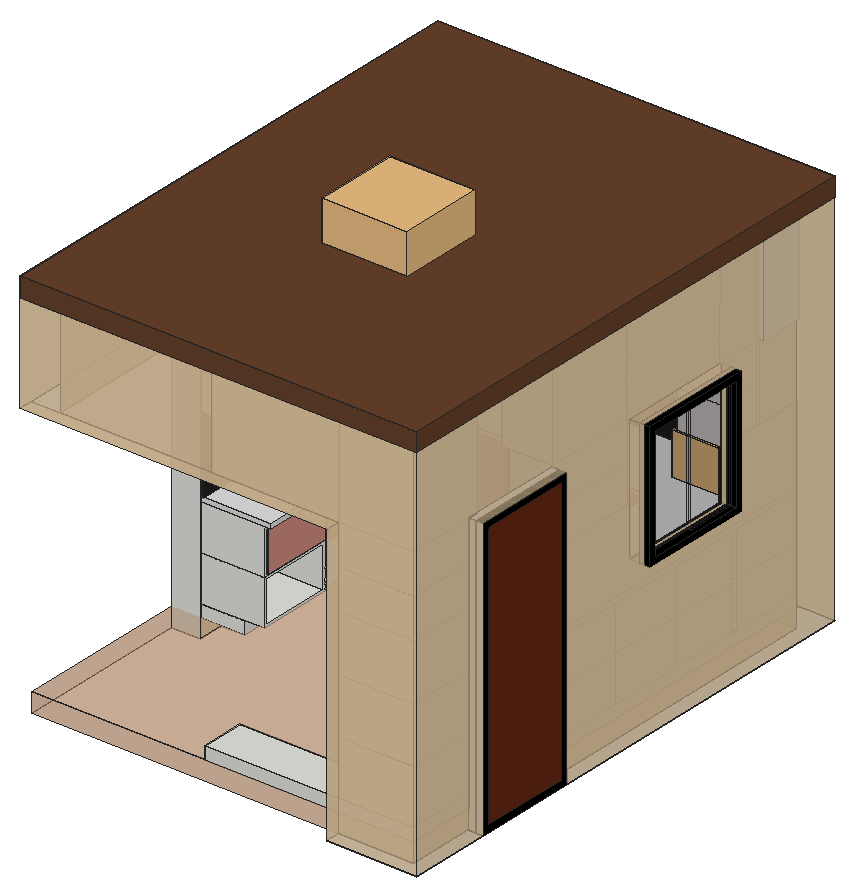
# SketchUp Ruby script. Lengths in inches.
U = 1.inch
M = Sketchup.active_model
def pt(a) = Geom::Point3d.new(a.map { |v| v * U })
def face(e, loops, mat)
  f = e.add_face(loops[0].map { |a| pt(a) })
  loops[1..].each { |l| e.add_face(l.map { |a| pt(a) }).erase! }
  f.material = f.back_material = mat if mat
  f
end
# faces: each face lists its corners as indices into pts; further lists are holes
def faces(e, pts, list, mat = nil) = list.each { |f| face(e, (f[0].is_a?(Array) ? f : [f]).map { |l| l.map { |i| pts[i] } }, mat) }
# xy, xz, yz: faces in a plane at the given z, y or x. An outline is a flat list of corners, or four numbers for a rectangle; further outlines are holes
def ring(l) = l.size == 4 ? [[l[0], l[1]], [l[2], l[1]], [l[2], l[3]], [l[0], l[3]]] : l.each_slice(2).to_a
def flat(e, list, mat, &to3) = list.each { |f| face(e, (f[0].is_a?(Array) ? f : [f]).map { |l| ring(l).map { |u, v| to3.(u, v) } }, mat) }
def xy(e, z, list, mat = nil) = flat(e, list, mat) { |x, y| [x, y, z] }
def xz(e, y, list, mat = nil) = flat(e, list, mat) { |x, z| [x, y, z] }
def yz(e, x, list, mat = nil) = flat(e, list, mat) { |y, z| [x, y, z] }
def lines(e, pts, list) = list.each { |a, b| e.add_line(pt(pts[a]), pt(pts[b])) }
# prism: a flat outline (further loops are holes) pulled along v
def prism(e, loops, v, mat = nil)
  f = face(e, loops, mat); d = Geom::Vector3d.new(v.map { |x| x * U })
  f.pushpull(f.normal.samedirection?(d) ? d.length : -d.length)
end
def box(e, o, s, mat = nil) = prism(e, [[o, [o[0] + s[0], o[1], o[2]], [o[0] + s[0], o[1] + s[1], o[2]], [o[0], o[1] + s[1], o[2]]]], [0, 0, s[2]], mat)
def at(x, y, z, deg = 0) = Geom::Transformation.translation(pt([x, y, z])) * Geom::Transformation.rotation(ORIGIN, Z_AXIS, deg.degrees)
def axes(o, x, y, z) = Geom::Transformation.new([*x, 0, *y, 0, *z, 0, *pt(o).to_a, 1])
def part(name) = M.definitions.add(name)
# library, detail: a bought-in or finely detailed component or shape, given as its bounding box
def library(name, o, s) = part(name).tap { |d| box(d.entities, o, s) }
def detail(e, o, s) = box(e.add_group.entities, o, s)
def put(e, d, t, mat = nil) = e.add_instance(d, t).tap { |i| i.material = mat if mat }
def group(e, t, mat = nil) = e.add_group.tap { |g| g.transformation = t; g.material = mat if mat }.entities
root = M.entities
M.materials.add("BEIGE FOR CUPBOARDS").color = [205, 139, 125]
M.materials.add("Chocolate White WALL PAINT").color = [230, 202, 161]
M.materials["Chocolate White WALL PAINT"].alpha = 0.75
M.materials.add("GLASS").color = [0, 0, 0]
M.materials["GLASS"].alpha = 0.1
M.materials.add("METAL").color = [0, 0, 0]
M.materials.add("Marble Black 100cm").color = [32, 32, 32]
M.materials.add("Marble White SSS 100cm").color = [222, 222, 222]
M.materials.add("Onyx 100cm").color = [192, 149, 115]
M.materials["Onyx 100cm"].alpha = 0.47
M.materials.add("Roof Ceramic 22-10 200cm").color = [102, 65, 42]
M.materials.add("WHITE  FOR CUPBOARDS").color = [218, 213, 212]
M.materials.add("Wood Dark 02 100cm").color = [99, 39, 19]
M.materials["Wood Dark 02 100cm"].alpha = 0.97
c1 = library("Cutlery Box 145 009",[-8.61,-2.8,0],[17.18,6.16,8.82])
c2 = library("Spice Stand 145 027",[-6.18,-5.51,0],[12.36,11.02,14.15])
c3 = library("Breakfast Meal Set 145 006",[-7.73,-8.125,0],[15.46,19.06,8.53])
c4 = library("Kitchen Props 134 014",[-15.6875,-7.04,0],[31.37,14.09,12.97])
c5 = library("Sphere Light",[-13.29,-13.29,-13.29],[26.58,26.58,26.58])
c6 = library("Spot Light",[-5.1,-5.1,-11.05],[10.2,10.2,11.05])
c7 = library("Spot Light\#1",[-5.1,-5.1,-11.05],[10.2,10.2,11.05])
c8 = library("Spot Light\#2",[-5.1,-5.1,-11.05],[10.2,10.2,11.05])
c9 = library("Spot Light\#3",[-5.1,-5.1,-11.05],[10.2,10.2,11.05])
c10 = part("Group\#20")
xy(c10.entities,0,[[0,-2.26,23.62,21.36]])
xy(c10.entities,0.81,[[0,-1.45,22.05,20.56]])
xy(c10.entities,13.37,[[0,-1.45,22.05,20.56]])
xy(c10.entities,14.17,[[0,-2.26,23.62,21.36]])
xz(c10.entities,-2.26,[[0,0,23.62,14.17]])
xz(c10.entities,-1.45,[[0,0.81,22.05,13.37]])
xz(c10.entities,20.56,[[0,0.81,22.05,13.37]])
xz(c10.entities,21.36,[[0,0,23.62,14.17]])
yz(c10.entities,0,[[[-2.16,0.1,21.26,14.07],[-1.45,0.81,20.56,13.37]]])
yz(c10.entities,22.05,[[-1.45,0.81,20.56,13.37]])
yz(c10.entities,23.62,[[-2.26,0,21.36,14.17]])
c11 = part("Group\#23")
box(c11.entities,[-0.71,0,0],[0.71,22.01,12.56])
c12 = part("Group\#40")
xy(c12.entities,0,[[0,-1.97,19.78,21.65]])
xy(c12.entities,0.71,[[4.04,-1.26,19.78,20.94]])
xy(c12.entities,13.46,[[4.04,-1.26,19.78,20.94]])
xy(c12.entities,14.17,[[0,-1.97,19.78,21.65]])
xz(c12.entities,-1.97,[[0,0,19.78,14.17]])
xz(c12.entities,-1.26,[[4.04,0.71,19.78,13.46]])
xz(c12.entities,20.94,[[4.04,0.71,19.78,13.46]])
xz(c12.entities,21.65,[[0,0,19.78,14.17]])
yz(c12.entities,0,[[-1.97,0,21.65,14.17]])
yz(c12.entities,4.04,[[-1.26,0.71,20.94,13.46]])
yz(c12.entities,19.78,[[[-1.87,0.1,21.56,14.07],[-1.26,0.71,20.94,13.46]]])
c13 = part("Group\#43")
box(c13.entities,[0,0,0],[0.71,22.01,12.56])
c14 = part("Group\#24")
box(c14.entities,[0,-2.26,0],[23.62,23.62,14.17])
c15 = part("Group\#82")
box(c15.entities,[0,-0.71,0],[13.35,0.71,10.2])
c16 = part("Group\#62")
box(c16.entities,[-0.71,0,0],[0.71,17.3,27.91])
c17 = part("Group\#79")
box(c17.entities,[0,1,-0.35],[6.26,10.8125,0.7])
c18 = part("Group\#63")
box(c18.entities,[-0.71,0,0],[0.71,13.86,28.11])
c19 = part("Group\#84")
box(c19.entities,[0,-0.71,0],[13.54,0.71,28.11])
c20 = part("Group\#92")
box(c20.entities,[0,0,0],[0.71,22.01,10.2])
c21 = part("Group\#93")
box(c21.entities,[0,0,0],[0.71,22.2,28.11])
p = [[119.24,25.58,0],[123.74,25.58,0]]
lines(root,p,[[0,1]])
put(root,c1,at(19.45,148.53,39.86))
put(root,c2,at(16.11,131.18,39.85,90))
put(root,c3,at(21.28,114.77,39.86,-180))
put(root,c4,axes([105.33,146.65,39.86],[0.82,0,0],[0,1.17,0],[0,0,1]))
put(root,c5,at(60.16,72.25,123.27))
put(root,c6,at(30.14,28.18,118.19))
put(root,c7,at(93.57,127.28,118.19))
put(root,c8,at(29.38,127.67,118.19))
put(root,c9,at(102.72,34.74,118.19))
g1 = group(root,at(0,0,0))
g2 = group(g1,at(0,0,0))
g3 = group(g2,at(0,0,0))
g4 = group(g3,at(9,106.47,24.11))
xy(g4,0,[[0,0,19.78,21.65]])
xy(g4,0.81,[[4.04,0.81,19.78,20.85]])
xy(g4,13.37,[[4.04,0.81,19.78,20.85]])
xy(g4,14.17,[[0,0,19.78,21.65]])
xz(g4,0,[[0,0,19.78,14.17]])
xz(g4,0.81,[[4.04,0.81,19.78,13.37]])
xz(g4,20.85,[[4.04,0.81,19.78,13.37]])
xz(g4,21.65,[[0,0,19.78,14.17]])
yz(g4,0,[[0,0,21.65,14.17]])
yz(g4,4.04,[[0.81,0.81,20.85,13.37]])
yz(g4,19.78,[[[0.1,0.1,21.56,14.07],[0.81,0.81,20.85,13.37]]])
g5 = group(g3,at(9,4.5,9.9375))
put(g5,c10,at(86.61,56.98,0))
g6 = group(g5,at(86.61,56.98,14.17))
xy(g6,0,[[0,-2.26,23.62,21.36]])
xy(g6,0.81,[[0,-1.45,22.05,20.56]])
xy(g6,13.37,[[0,-1.45,22.05,20.56]])
xy(g6,14.17,[[0,-2.26,23.62,21.36]])
xz(g6,-2.26,[[0,0,23.62,14.17]])
xz(g6,-1.45,[[0,0.81,22.05,13.37]])
xz(g6,20.56,[[0,0.81,22.05,13.37]])
xz(g6,21.36,[[0,0,23.62,14.17]])
yz(g6,0,[[[-2.16,0.1,21.26,14.07],[-1.45,0.81,20.56,13.37]]])
yz(g6,22.05,[[-1.45,0.81,20.56,13.37]])
yz(g6,23.62,[[-2.26,0,21.36,14.17]])
put(g6,c11,at(0,-1.45,0.81),"BEIGE FOR CUPBOARDS")
g7 = group(g5,at(86.61,0,17.22),"WHITE  FOR CUPBOARDS")
xy(g7,0,[[0,0,23.62,24.56]])
xy(g7,0.71,[[0.71,4.875,22.91,24.56]])
xy(g7,16.52,[[0.71,4.875,22.91,24.56]])
xy(g7,17.22,[[0,0,23.62,24.56]])
xz(g7,0,[[0,0,23.62,17.22]])
xz(g7,4.875,[[0.71,0.71,22.91,16.52]])
xz(g7,24.56,[[[0.1,0.1,23.52,17.125],[0.71,0.71,22.91,16.52]]])
yz(g7,0,[[0,0,24.56,17.22]])
yz(g7,0.71,[[4.875,0.71,24.56,16.52]])
yz(g7,22.91,[[4.875,0.71,24.56,16.52]])
yz(g7,23.62,[[0,0,24.56,17.22]])
g8 = group(g5,at(86.61,0,0),"WHITE  FOR CUPBOARDS")
xy(g8,0,[[0,0,23.62,24.56]])
xy(g8,0.81,[[0.81,4.75,22.81,24.56]])
xy(g8,16.42,[[0.81,4.75,22.81,24.56]])
xy(g8,17.22,[[0,0,23.62,24.56]])
xz(g8,0,[[0,0,23.62,17.22]])
xz(g8,4.75,[[0.81,0.81,22.81,16.42]])
xz(g8,24.56,[[[0.1,0.1,23.52,17.125],[0.81,0.81,22.81,16.42]]])
yz(g8,0,[[0,0,24.56,17.22]])
yz(g8,0.81,[[4.75,0.81,24.56,16.42]])
yz(g8,22.81,[[4.75,0.81,24.56,16.42]])
yz(g8,23.62,[[0,0,24.56,17.22]])
g9 = group(g5,at(86.61,0,52.17),"WHITE  FOR CUPBOARDS")
xy(g9,0,[[0,0,23.62,24.56]])
xy(g9,0.81,[[0.81,4.875,22.81,24.56]])
xy(g9,11.69,[[0.81,4.875,22.81,24.56]])
xy(g9,12.5,[[0,0,23.62,24.56]])
xz(g9,0,[[0,0,23.62,12.5]])
xz(g9,4.875,[[0.81,0.81,22.81,11.69]])
xz(g9,24.56,[[[0.1,0.1,23.52,12.4],[0.81,0.81,22.81,11.69]]])
yz(g9,0,[[0,0,24.56,12.5]])
yz(g9,0.81,[[4.875,0.81,24.56,11.69]])
yz(g9,22.81,[[4.875,0.81,24.56,11.69]])
yz(g9,23.62,[[0,0,24.56,12.5]])
g10 = group(g5,at(86.61,0,77.17))
xy(g10,0,[[0,0,23.62,24.56]],"WHITE  FOR CUPBOARDS")
xy(g10,29.53,[[0,0,23.62,24.56]],"WHITE  FOR CUPBOARDS")
xz(g10,0,[[0,0,23.62,29.53]],"WHITE  FOR CUPBOARDS")
yz(g10,0,[[0,0,24.56,29.53]],"WHITE  FOR CUPBOARDS")
yz(g10,23.62,[[0,0,24.56,29.53]],"WHITE  FOR CUPBOARDS")
g11 = group(g10,at(0.1,4.875,0.1),"BEIGE FOR CUPBOARDS")
xy(g11,0.71,[[0.71,0,22.72,19.69],[0.71,19.69,22.72,20.39]])
xy(g11,28.62,[[0.71,0,22.72,19.69],[0.71,19.69,22.72,20.39]])
xz(g11,0,[[0.71,0.71,22.72,28.62]])
xz(g11,19.69,[[[0,0,23.43,29.33],[0.71,0.71,22.72,28.62]]],"WHITE  FOR CUPBOARDS")
xz(g11,20.39,[[0.71,0.71,22.72,28.62]])
yz(g11,0.71,[[0,0.71,19.69,28.62],[19.69,0.71,20.39,28.62]])
yz(g11,22.72,[[0,0.71,19.69,28.62],[19.69,0.71,20.39,28.62]])
g12 = group(g5,at(86.61,0,34.45),"WHITE  FOR CUPBOARDS")
xy(g12,0,[[0,0,23.62,24.56]])
xy(g12,0.81,[[0.81,4.875,22.81,24.56]])
xy(g12,16.91,[[0.81,4.875,22.81,24.56]])
xy(g12,17.72,[[0,0,23.62,24.56]])
xz(g12,0,[[0,0,23.62,17.72]])
xz(g12,4.875,[[0.81,0.81,22.81,16.91]])
xz(g12,24.56,[[[0.1,0.1,23.52,17.62],[0.81,0.81,22.81,16.91]]])
yz(g12,0,[[0,0,24.56,17.72]])
yz(g12,0.81,[[4.875,0.81,24.56,16.91]])
yz(g12,22.81,[[4.875,0.81,24.56,16.91]])
yz(g12,23.62,[[0,0,24.56,17.72]])
g13 = group(g5,at(62.99,0,77.17))
xy(g13,0,[[-15.75,0,23.62,24.56]],"WHITE  FOR CUPBOARDS")
xy(g13,0.81,[[-14.94,4.875,22.81,24.56]])
xy(g13,28.72,[[-14.94,4.875,22.81,24.56]])
xy(g13,29.53,[[-15.75,0,23.62,24.56]],"WHITE  FOR CUPBOARDS")
xz(g13,0,[[-15.75,0,23.62,29.53]],"WHITE  FOR CUPBOARDS")
xz(g13,4.875,[[-14.94,0.81,22.81,28.72]])
xz(g13,24.56,[[[-15.65,0.1,23.52,29.43],[-14.94,0.81,22.81,28.72]]],"WHITE  FOR CUPBOARDS")
yz(g13,-15.75,[[0,0,24.56,29.53]],"WHITE  FOR CUPBOARDS")
yz(g13,-14.94,[[4.875,0.81,24.56,28.72]])
yz(g13,22.81,[[4.875,0.81,24.56,28.72]])
yz(g13,23.62,[[0,0,24.56,29.53]],"WHITE  FOR CUPBOARDS")
g14 = group(g13,at(3.9375,24.56,0.81),"BEIGE FOR CUPBOARDS")
box(g14,[0,0,0],[18.88,0.71,27.91])
g15 = group(g13,at(-14.94,24.56,0.81),"BEIGE FOR CUPBOARDS")
box(g15,[0,0,0],[18.88,0.71,27.91])
g16 = group(g5,at(86.61,0,64.67))
xy(g16,0,[[0,0,23.62,24.56]],"WHITE  FOR CUPBOARDS")
xy(g16,0.71,[[0.71,4.875,22.91,24.56]])
xy(g16,11.79,[[0.71,4.875,22.91,24.56]])
xy(g16,12.5,[[0,0,23.62,24.56]],"WHITE  FOR CUPBOARDS")
xz(g16,0,[[0,0,23.62,12.5]],"WHITE  FOR CUPBOARDS")
xz(g16,4.875,[[0.71,0.71,22.91,11.79]])
xz(g16,24.56,[[[0.1,0.1,23.52,12.4],[0.71,0.71,22.91,11.79]]],"WHITE  FOR CUPBOARDS")
yz(g16,0,[[0,0,24.56,12.5]],"WHITE  FOR CUPBOARDS")
yz(g16,0.71,[[4.875,0.71,24.56,11.79]])
yz(g16,22.91,[[4.875,0.71,24.56,11.79]])
yz(g16,23.62,[[0,0,24.56,12.5]],"WHITE  FOR CUPBOARDS")
g17 = group(g16,at(0.71,24.56,0.71),"BEIGE FOR CUPBOARDS")
box(g17,[0,0,0],[22.2,0.71,11.08])
g18 = group(g5,at(87.32,24.56,17.93))
box(g18,[0,0,0],[22.2,0.71,15.81],"BEIGE FOR CUPBOARDS")
put(g5,c12,at(0,80.31,0))
g19 = group(g5,at(0,80.31,14.17))
xy(g19,0,[[0,-1.97,19.78,21.65]])
xy(g19,0.81,[[4.04,-1.16,19.78,20.85]])
xy(g19,13.37,[[4.04,-1.16,19.78,20.85]])
xy(g19,14.17,[[0,-1.97,19.78,21.65]])
xz(g19,-1.97,[[0,0,19.78,14.17]])
xz(g19,-1.16,[[4.04,0.81,19.78,13.37]])
xz(g19,20.85,[[4.04,0.81,19.78,13.37]])
xz(g19,21.65,[[0,0,19.78,14.17]])
yz(g19,0,[[-1.97,0,21.65,14.17]])
yz(g19,4.04,[[-1.16,0.81,20.85,13.37]])
yz(g19,19.78,[[[-1.87,0.1,21.56,14.07],[-1.16,0.81,20.85,13.37]]])
put(g19,c13,at(19.78,-1.16,0.81),"BEIGE FOR CUPBOARDS")
g20 = group(g5,at(0,125.59,0))
box(g20,[0,0,0],[17.72,23.62,28.35])
g21 = group(g5,at(0,101.97,0))
xy(g21,0,[[0,0,19.78,21.65]])
xy(g21,0.81,[[4.04,0.81,19.78,20.85]])
xy(g21,13.37,[[4.04,0.81,19.78,20.85]])
xy(g21,14.17,[[0,0,19.78,21.65]])
xz(g21,0,[[0,0,19.78,14.17]])
xz(g21,0.81,[[4.04,0.81,19.78,13.37]])
xz(g21,20.85,[[4.04,0.81,19.78,13.37]])
xz(g21,21.65,[[0,0,19.78,14.17]])
yz(g21,0,[[0,0,21.65,14.17]])
yz(g21,4.04,[[0.81,0.81,20.85,7.09],[0.81,7.09,20.85,13.37]])
yz(g21,19.78,[[[0,0,21.65,14.17],[0.1,0.1,21.56,14.07]],[[0.1,0.1,21.56,14.07],[0.81,0.81,20.85,13.37]]])
g22 = group(g21,at(4.04,0.81,7.09))
box(g22,[0,0,-0.35],[13.75,20.04,0.7])
g23 = group(g5,at(0,56.69,14.17))
xy(g23,0,[[0,-1.97,19.78,21.65]])
xy(g23,0.81,[[4.04,-1.16,19.78,20.85]])
xy(g23,13.37,[[4.04,-1.16,19.78,20.85]])
xy(g23,14.17,[[0,-1.97,19.78,21.65]])
xz(g23,-1.97,[[0,0,19.78,14.17]])
xz(g23,-1.16,[[4.04,0.81,19.78,13.37]])
xz(g23,20.85,[[4.04,0.81,19.78,13.37]])
xz(g23,21.65,[[0,0,19.78,14.17]])
yz(g23,0,[[-1.97,0,21.65,14.17]])
yz(g23,4.04,[[-1.16,0.81,20.85,13.37]])
yz(g23,19.78,[[[-1.87,0.1,21.56,14.07],[-1.16,0.81,20.85,13.37]]])
put(g23,c13,at(19.78,-1.16,0.81),"BEIGE FOR CUPBOARDS")
put(g5,c12,at(0,56.69,0))
g24 = group(g5,at(19.78,102.78,14.98),"BEIGE FOR CUPBOARDS")
box(g24,[0,0,0],[0.71,20.04,12.56])
g25 = group(g5,at(55.12,125.59,23.03))
xy(g25,0,[[0,0,23.62,23.62]])
xy(g25,0.81,[[0.81,0,22.81,22.05]])
xy(g25,4.51,[[0.81,0,22.81,22.05]])
xy(g25,5.3125,[[0,0,23.62,23.62]])
xz(g25,0,[[[0.1,0.1,23.52,5.21],[0.81,0.81,22.81,4.51]]])
xz(g25,22.05,[[0.81,0.81,22.81,4.51]])
xz(g25,23.62,[[0,0,23.62,5.3125]])
yz(g25,0,[[0,0,23.62,5.3125]])
yz(g25,0.81,[[0,0.81,22.05,4.51]])
yz(g25,22.81,[[0,0.81,22.05,4.51]])
yz(g25,23.62,[[0,0,23.62,5.3125]])
g26 = group(g25,at(0.81,0,0.81),"BEIGE FOR CUPBOARDS")
box(g26,[0,-0.71,0],[22.01,0.71,3.7])
put(g5,c14,at(107.98,125.59,0,90))
g27 = group(g5,at(55.12,125.59,0))
xy(g27,0,[[0,0,23.62,23.62]])
xy(g27,0.71,[[0.71,0,22.91,22.05]])
xy(g27,13.07,[[0.71,0,22.91,22.05]])
xy(g27,13.78,[[0,0,23.62,23.62]])
xz(g27,0,[[[0.1,0.1,23.52,13.68],[0.71,0.71,22.91,13.07]]])
xz(g27,22.05,[[0.71,0.71,22.91,13.07]])
xz(g27,23.62,[[0,0,23.62,13.78]])
yz(g27,0,[[0,0,23.62,13.78]])
yz(g27,0.71,[[0,0.71,22.05,13.07]])
yz(g27,22.91,[[0,0.71,22.05,13.07]])
yz(g27,23.62,[[0,0,23.62,13.78]])
g28 = group(g27,at(0.71,0,0.71),"BEIGE FOR CUPBOARDS")
box(g28,[0,-0.71,0],[22.2,0.71,12.36])
g29 = group(g5,at(19.69,125.59,0))
xy(g29,0,[[0,0,19.69,23.62]])
xy(g29,0.81,[[0.81,0,18.88,22.05]])
xy(g29,27.54,[[0.81,0,18.88,22.05]])
xy(g29,28.35,[[0,0,19.69,23.62]])
xz(g29,0,[[[0.1,0.1,19.59,28.25],[0.81,0.81,18.88,27.54]]])
xz(g29,22.05,[[0.81,0.81,18.88,27.54]])
xz(g29,23.62,[[0,0,19.69,28.35]])
yz(g29,0,[[0,0,23.62,28.35]])
yz(g29,0.81,[[0,0.81,22.05,27.54]])
yz(g29,18.88,[[0,0.81,22.05,27.54]])
yz(g29,19.69,[[0,0,23.62,28.35]])
g30 = group(g29,at(0.81,0,0.81),"BEIGE FOR CUPBOARDS")
box(g30,[0,-0.71,0],[18.07,0.71,26.73])
g31 = group(g5,at(78.74,125.59,0))
xy(g31,0,[[0,0,5.91,23.62]])
xy(g31,0.71,[[0.71,0,5.2,22.05]])
xy(g31,27.64,[[0.71,0,5.2,22.05]])
xy(g31,28.35,[[0,0,5.91,23.62]])
xz(g31,0,[[[0.1,0.1,5.81,28.25],[0.71,0.71,5.2,27.64]]])
xz(g31,22.05,[[0.71,0.71,5.2,27.64]])
xz(g31,23.62,[[0,0,5.91,28.35]])
yz(g31,0,[[0,0,23.62,28.35]])
yz(g31,0.71,[[0,0.71,22.05,27.64]])
yz(g31,5.2,[[0,0.71,22.05,27.64]])
yz(g31,5.91,[[0,0,23.62,28.35]])
g32 = group(g31,at(0.71,0,0.71),"BEIGE FOR CUPBOARDS")
box(g32,[0,-0.71,0],[4.49,0.71,26.93])
g33 = group(g5,at(39.37,125.59,0))
xy(g33,0,[[0,0,15.75,23.62]])
xy(g33,0.81,[[0.81,0,14.94,22.05]])
xy(g33,12.97,[[0.81,0,14.94,22.05]])
xy(g33,13.78,[[0,0,15.75,23.62]])
xz(g33,0,[[[0.1,0.1,15.65,13.68],[0.81,0.81,14.94,12.97]]])
xz(g33,22.05,[[0.81,0.81,14.94,12.97]])
xz(g33,23.62,[[0,0,15.75,13.78]])
yz(g33,0,[[0,0,23.62,13.78]])
yz(g33,0.81,[[0,0.81,22.05,12.97]])
yz(g33,14.94,[[0,0.81,22.05,12.97]])
yz(g33,15.75,[[0,0,23.62,13.78]])
g34 = group(g5,at(55.12,125.59,14.57))
xy(g34,0,[[0,0,23.62,23.62]])
xy(g34,8.47,[[0,0,23.62,23.62]])
xz(g34,0,[[0.1,0.1,23.52,8.37]])
xz(g34,23.62,[[0,0,23.62,8.47]])
yz(g34,0,[[0,0,23.62,8.47]])
yz(g34,23.62,[[0,0,23.62,8.47]])
g35 = group(g34,at(0.81,0,0.81),"BEIGE FOR CUPBOARDS")
box(g35,[0,-0.71,0],[22.01,0.71,6.85])
g36 = group(g5,at(39.37,125.59,14.57))
xy(g36,0,[[0,0,15.75,23.62]])
xy(g36,0.81,[[0.81,0,14.94,22.05]])
xy(g36,12.97,[[0.81,0,14.94,22.05]])
xy(g36,13.78,[[0,0,15.75,23.62]])
xz(g36,0,[[[0.1,0.1,15.65,13.68],[0.81,0.81,14.94,12.97]]])
xz(g36,22.05,[[0.81,0.81,14.94,12.97]])
xz(g36,23.62,[[0,0,15.75,13.78]])
yz(g36,0,[[0,0,23.62,13.78]])
yz(g36,0.81,[[0,0.81,22.05,12.97]])
yz(g36,14.94,[[0,0.81,22.05,12.97]])
yz(g36,15.75,[[0,0,23.62,13.78]])
g37 = group(g36,at(0.81,0,0.81),"BEIGE FOR CUPBOARDS")
box(g37,[0,-0.71,0],[14.13,0.71,12.17])
g38 = group(g5,at(86.61,101.97,14.17))
xy(g38,0,[[0,0,23.62,21.36]])
xy(g38,0.81,[[0,0.81,22.11,20.56]])
xy(g38,13.37,[[0,0.81,22.11,20.56]])
xy(g38,14.17,[[0,0,23.62,21.36]])
xz(g38,0,[[0,0,23.62,14.17]])
xz(g38,0.81,[[0,0.81,22.11,13.37]])
xz(g38,20.56,[[0,0.81,22.11,13.37]])
xz(g38,21.36,[[0,0,23.62,14.17]])
yz(g38,0,[[[0.1,0.1,21.26,14.07],[0.81,0.81,20.56,13.37]]])
yz(g38,22.11,[[0.81,0.81,20.56,13.37]])
yz(g38,23.62,[[0,0,21.36,14.17]])
g39 = group(g38,at(0,0.81,0.81),"BEIGE FOR CUPBOARDS")
box(g39,[-0.71,0,0],[0.71,19.75,12.56])
g40 = group(g5,at(86.61,101.97,0))
xy(g40,0,[[0,0,23.62,21.36]])
xy(g40,0.81,[[0,0.81,22.05,20.56]])
xy(g40,13.37,[[0,0.81,22.05,20.56]])
xy(g40,14.17,[[0,0,23.62,21.36]])
xz(g40,0,[[0,0,23.62,14.17]])
xz(g40,0.81,[[0,0.81,22.05,13.37]])
xz(g40,20.56,[[0,0.81,22.05,13.37]])
xz(g40,21.36,[[0,0,23.62,14.17]])
yz(g40,0,[[[0.1,0.1,21.26,14.07],[0.81,0.81,20.56,13.37]]])
yz(g40,22.05,[[0.81,0.81,20.56,7.09],[0.81,7.09,20.56,13.37]])
yz(g40,23.62,[[0,0,21.36,14.17]])
g41 = group(g40,at(0,0.81,7.09))
box(g41,[2,0,-0.35],[20.05,19.75,0.7])
put(g5,c10,at(86.61,80.61,0))
g42 = group(g5,at(86.61,80.61,14.17))
xy(g42,0,[[0,-2.26,23.62,21.36]])
xy(g42,0.81,[[0,-1.45,22.05,20.56]])
xy(g42,13.37,[[0,-1.45,22.05,20.56]])
xy(g42,14.17,[[0,-2.26,23.62,21.36]])
xz(g42,-2.26,[[0,0,23.62,14.17]])
xz(g42,-1.45,[[0,0.81,22.05,13.37]])
xz(g42,20.56,[[0,0.81,22.05,13.37]])
xz(g42,21.36,[[0,0,23.62,14.17]])
yz(g42,0,[[[-2.16,0.1,21.26,14.07],[-1.45,0.81,20.56,13.37]]])
yz(g42,22.05,[[-1.45,0.81,20.56,13.37]])
yz(g42,23.62,[[-2.26,0,21.36,14.17]])
put(g42,c11,at(0,-1.45,0.81),"BEIGE FOR CUPBOARDS")
put(g5,c14,at(107.98,125.59,14.17,90))
g43 = group(g3,at(0,0,6))
box(g43,[0,4.5,-6],[119.24,149.21,6],"Onyx 100cm")
g44 = group(g3,at(9,4.5,6))
prism(g44,[[[0,54.72,0],[0,149.21,0],[110.24,149.21,0],[110.24,54.72,0],[96.46,54.72,0],[96.46,135.43,0],[13.78,135.43,0],[13.78,54.72,0]]],[0,0,3.9375])
prism(g44,[[[96.46,13.78,0],[96.46,21.46,0],[110.24,21.46,0],[110.24,0,0],[44.93,0,0],[44.93,13.78,0]]],[0,0,3.9375])
g45 = group(g3,at(9,4.5,38.28),"Marble White SSS 100cm")
prism(g45,[[[0,54.72,0],[0,149.21,0],[110.24,149.21,0],[110.24,54.72,0],[84.61,54.72,0],[84.61,123.59,0],[21.78,123.59,0],[21.78,54.72,0]]],[0,0,1.57],"Marble White SSS 100cm")
g46 = group(g3,at(119.24,59.22,39.86))
xy(g46,0,[[-1,0,0,94.49]])
xy(g46,7.875,[[0,29.53,0,65.36,-1,65.36,-1,29.68]],"Marble Black 100cm")
xy(g46,23.62,[[-1,65.36,0,94.49]])
xy(g46,23.62,[[-1,0,0,0,0,29.53,-1,29.68]],"Marble Black 100cm")
xz(g46,0,[[-1,0,0,23.62]],"Marble Black 100cm")
xz(g46,65.36,[[-1,7.875,0,23.62]],"Marble Black 100cm")
xz(g46,94.49,[[-1,0,0,23.62]])
yz(g46,-1,[[0,0,0,23.62,29.68,23.62,29.68,7.875,65.36,7.875,65.36,23.62,94.49,23.62,94.49,0]],"Marble Black 100cm")
yz(g46,0,[[0,0,94.49,0,94.49,23.62,65.36,23.62,65.36,7.875,29.53,7.875,29.53,23.62,0,23.62]])
p = [[-1,29.68,23.62],[0,29.53,23.62],[0,29.53,7.875],[-1,29.68,7.875]]
faces(g46,p,[[0,1,2,3]],"Marble Black 100cm")
g47 = group(g2,at(0,0,0))
xy(g47,0,[[95.61,0,95.61,4.5,119.24,4.5,119.24,25.96,123.74,25.96,123.74,0],[119.24,58.4375,119.24,153.71,9,153.71,9,59.22,0,59.22,0,162.71,123.74,162.71,123.74,58.4375]])
xy(g47,47.73,[[119.24,88.75,123.74,124.58]],"Chocolate White WALL PAINT")
xy(g47,87,[[0,0,95.61,4.5]],"Chocolate White WALL PAINT")
xy(g47,87.1,[[0,4.5,9,59.22],[119.24,25.96,123.74,58.4375]])
xy(g47,87.1,[[119.24,88.75,123.74,124.58]],"Chocolate White WALL PAINT")
xy(g47,118.2,[[[0,0,123.74,162.71],[9,4.5,119.24,153.71]]],"Chocolate White WALL PAINT")
xz(g47,0,[[95.61,0,123.74,0,123.74,118.2,0,118.2,0,87,95.61,87]],"Chocolate White WALL PAINT")
xz(g47,4.5,[[95.61,0,95.61,87,0,87,0,87.1,9,87.1,9,118.2,119.24,118.2,119.24,0]],"Chocolate White WALL PAINT")
xz(g47,25.96,[[119.24,0,123.74,87.1]])
xz(g47,58.4375,[[119.24,0,123.74,87.1]])
xz(g47,59.22,[[0,0,9,87.1]])
xz(g47,88.75,[[119.24,47.73,123.74,87.1]],"Chocolate White WALL PAINT")
xz(g47,124.58,[[119.24,47.73,123.74,87.1]],"Chocolate White WALL PAINT")
xz(g47,153.71,[[9,0,119.24,118.2]],"Chocolate White WALL PAINT")
xz(g47,162.71,[[0,0,123.74,118.2]],"Chocolate White WALL PAINT")
yz(g47,0,[[59.22,0,59.22,87.1,4.5,87.1,4.5,87,0,87,0,118.2,162.71,118.2,162.71,0]],"Chocolate White WALL PAINT")
yz(g47,9,[[59.22,0,153.71,0,153.71,118.2,4.5,118.2,4.5,87.1,59.22,87.1]],"Chocolate White WALL PAINT")
yz(g47,95.61,[[0,0,4.5,87]],"Chocolate White WALL PAINT")
yz(g47,119.24,[[[4.5,0,4.5,118.2,153.71,118.2,153.71,0,58.4375,0,58.4375,87.1,25.96,87.1,25.96,0],[88.75,47.73,124.58,87.1]]],"Chocolate White WALL PAINT")
yz(g47,123.74,[[[0,0,25.96,0,25.96,87.1,58.4375,87.1,58.4375,0,162.71,0,162.71,118.2,0,118.2],[88.75,47.73,124.58,87.1]]],"Chocolate White WALL PAINT")
g48 = group(g47,at(123.74,88.75,47.73))
xy(g48,0,[[-1.5,0,1.5,35.83]],"METAL")
xy(g48,2,[[-1.5,2,1.5,33.83]],"METAL")
xy(g48,37.37,[[-1.5,2,1.5,33.83]],"METAL")
xy(g48,39.37,[[-1.5,0,1.5,35.83]],"METAL")
xz(g48,0,[[-1.5,0,1.5,39.37]],"METAL")
xz(g48,2,[[-1.5,2,1.5,37.37]],"METAL")
xz(g48,33.83,[[-1.5,2,1.5,37.37]],"METAL")
xz(g48,35.83,[[-1.5,0,1.5,39.37]],"METAL")
yz(g48,-1.5,[[[0,0,35.83,39.37],[2,2,33.83,37.37]]],"METAL")
yz(g48,1.5,[[[0,0,35.83,39.37],[2,2,33.83,37.37]]],"METAL")
g49 = group(g48,at(-0.5625,2,2),"GLASS")
box(g49,[-0.71,0,0],[0.71,15.91,35.37])
g50 = group(g48,at(0.15,17.91,2))
box(g50,[-0.71,0,0],[0.71,15.91,35.37],"GLASS")
g51 = group(g47,at(123.74,25.96,0),"METAL")
prism(g51,[[[0,32.48,0],[0,32.48,87.1],[0,0,87.1],[0,0,0]],[[0,30.48,85.1],[0,30.48,2],[0,2,2],[0,2,85.1]]],[-2.5,0,0])
g52 = group(g2,at(9,153.71,39.86))
box(g52,[0,-1,0],[109.24,1,23.62],"Marble Black 100cm")
g53 = group(g2,at(9,59.22,39.86))
box(g53,[0,0,0],[1,93.49,23.62],"Marble Black 100cm")
g54 = group(g1,at(9,58.4375,63.75))
g55 = group(g54,at(39.37,94.49,11.8125))
xy(g55,0,[[0,-12.81,14.96,0]],"WHITE  FOR CUPBOARDS")
xy(g55,0.81,[[0.81,-12.81,14.15,-3.2]],"WHITE  FOR CUPBOARDS")
xy(g55,11,[[0.81,-12.81,14.15,-3.2]],"WHITE  FOR CUPBOARDS")
xy(g55,11.8125,[[0,-12.81,14.96,0]],"WHITE  FOR CUPBOARDS")
xz(g55,-12.81,[[[0,0,14.96,11.8125],[0.1,0.1,14.86,11.71]],[[0.1,0.1,14.86,11.71],[0.81,0.81,14.15,11]]],"WHITE  FOR CUPBOARDS")
xz(g55,-3.2,[[0.81,0.81,14.15,11]],"WHITE  FOR CUPBOARDS")
xz(g55,0,[[0,0,14.96,11.8125]],"WHITE  FOR CUPBOARDS")
yz(g55,0,[[-12.81,0,0,11.8125]],"WHITE  FOR CUPBOARDS")
yz(g55,0.81,[[-12.81,0.81,-3.2,11]],"WHITE  FOR CUPBOARDS")
yz(g55,14.15,[[-12.81,0.81,-3.2,11]],"WHITE  FOR CUPBOARDS")
yz(g55,14.96,[[-12.81,0,0,11.8125]],"WHITE  FOR CUPBOARDS")
put(g55,c15,axes([0.81,-12.81,0.81],[1,0,0],[0,0.8134,0],[0,0,1]),"BEIGE FOR CUPBOARDS")
g56 = group(g54,at(39.37,94.49,0),"WHITE  FOR CUPBOARDS")
xy(g56,0,[[0,-12.81,14.96,0]])
xy(g56,0.71,[[0.71,-12.81,14.25,-3.15]])
xy(g56,11.1,[[0.71,-12.81,14.25,-3.15]])
xy(g56,11.8125,[[0,-12.81,14.96,0]])
xz(g56,-12.81,[[[0.1,0.1,14.86,11.71],[0.71,0.71,14.25,11.1]]])
xz(g56,-3.15,[[0.71,0.71,14.25,11.1]])
xz(g56,0,[[0,0,14.96,11.8125]])
yz(g56,0,[[-12.81,0,0,11.8125]])
yz(g56,0.71,[[-12.81,0.71,-3.15,11.1]])
yz(g56,14.25,[[-12.81,0.71,-3.15,11.1]])
yz(g56,14.96,[[-12.81,0,0,11.8125]])
g57 = group(g54,at(110.24,29.13,23.62))
xy(g57,0,[[-15.75,0,0,36.22]],"WHITE  FOR CUPBOARDS")
xy(g57,0.81,[[-15.75,0.81,-3.9375,35.41]])
xy(g57,28.72,[[-15.75,0.81,-3.9375,35.41]])
xy(g57,29.53,[[-15.75,0,0,36.22]],"WHITE  FOR CUPBOARDS")
xz(g57,0,[[-15.75,0,0,29.53]],"WHITE  FOR CUPBOARDS")
xz(g57,0.81,[[-15.75,0.81,-3.9375,28.72]])
xz(g57,35.41,[[-15.75,0.81,-3.9375,28.72]])
xz(g57,36.22,[[-15.75,0,0,29.53]],"WHITE  FOR CUPBOARDS")
yz(g57,-15.75,[[[0.1,0.1,36.12,29.43],[0.81,0.81,35.41,28.72]]],"WHITE  FOR CUPBOARDS")
yz(g57,-3.9375,[[0.81,0.81,35.41,28.72]])
yz(g57,0,[[0,0,36.22,29.53]],"WHITE  FOR CUPBOARDS")
put(g57,c16,at(-15.75,18.11,0.81),"BEIGE FOR CUPBOARDS")
put(g57,c16,at(-15.75,0.81,0.81),"BEIGE FOR CUPBOARDS")
g58 = group(g54,at(0,94.49,23.62),"WHITE  FOR CUPBOARDS")
box(g58,[0,-12.81,0],[13.78,12.81,29.53])
g59 = group(g54,at(110.24,65.35,23.62))
xy(g59,0,[[-15.75,0,0,13.78]],"WHITE  FOR CUPBOARDS")
xy(g59,0.71,[[-15.75,0.71,-3.9375,13.07]],"WHITE  FOR CUPBOARDS")
xy(g59,28.82,[[-15.75,0.71,-3.9375,13.07]],"WHITE  FOR CUPBOARDS")
xy(g59,29.53,[[-15.75,0,0,13.78]],"WHITE  FOR CUPBOARDS")
xz(g59,0,[[-15.75,0,0,29.53]],"WHITE  FOR CUPBOARDS")
xz(g59,0.71,[[-15.75,0.71,-3.9375,28.82]],"WHITE  FOR CUPBOARDS")
xz(g59,13.07,[[-15.75,0.71,-3.9375,28.82]],"WHITE  FOR CUPBOARDS")
xz(g59,13.78,[[-15.75,0,0,29.53]],"WHITE  FOR CUPBOARDS")
yz(g59,-15.75,[[[0.1,0.1,13.68,29.43],[0.71,0.71,13.07,28.82]]],"WHITE  FOR CUPBOARDS")
yz(g59,-3.9375,[[0.71,0.71,13.07,28.82]],"WHITE  FOR CUPBOARDS")
yz(g59,0,[[0,0,13.78,29.53]],"WHITE  FOR CUPBOARDS")
g60 = group(g59,at(-15.75,0.71,0.71),"BEIGE FOR CUPBOARDS")
box(g60,[-0.71,0,0],[0.71,12.36,28.11])
g61 = group(g54,at(13.78,94.49,11.8125),"WHITE  FOR CUPBOARDS")
xy(g61,0,[[0,-12.81,7.875,0]])
xy(g61,0.81,[[0.81,-12.81,7.07,-3.2]])
xy(g61,11,[[0.81,-12.81,7.07,-3.2]])
xy(g61,11.8125,[[0,-12.81,7.875,0]])
xz(g61,-12.81,[[[0.1,0.1,7.78,11.71],[0.81,0.81,7.07,11]]])
xz(g61,-3.2,[[0.81,0.81,7.07,5.91],[0.81,5.91,7.07,11]])
xz(g61,0,[[0,0,7.875,11.8125]])
yz(g61,0,[[-12.81,0,0,11.8125]])
yz(g61,0.81,[[-12.81,0.81,-3.2,11]])
yz(g61,7.07,[[-12.81,0.81,-3.2,11]])
yz(g61,7.875,[[-12.81,0,0,11.8125]])
put(g61,c17,axes([0.81,-12.81,5.91],[1,0,0],[0,0.8134,0],[0,0,1]))
g62 = group(g54,at(13.78,94.49,38.39),"WHITE  FOR CUPBOARDS")
xy(g62,0,[[0,-12.81,7.875,0]])
xy(g62,0.71,[[0.71,-12.81,7.17,-3.2]])
xy(g62,14.06,[[0.71,-12.81,7.17,-3.2]])
xy(g62,14.76,[[0,-12.81,7.875,0]],"WHITE  FOR CUPBOARDS")
xz(g62,-12.81,[[[0.1,0.1,7.78,14.67],[0.71,0.71,7.17,14.06]]])
xz(g62,-3.2,[[0.71,0.71,7.17,7.38],[0.71,7.38,7.17,14.06]])
xz(g62,0,[[0,0,7.875,14.76]])
yz(g62,0,[[-12.81,0,0,14.76]])
yz(g62,0.71,[[-12.81,0.71,-3.2,14.06]])
yz(g62,7.17,[[-12.81,0.71,-3.2,14.06]])
yz(g62,7.875,[[-12.81,0,0,14.76]])
g63 = group(g62,at(0.71,-12.81,7.38))
box(g63,[0,0.8125,-0.35],[6.46,8.8,0.7])
g64 = group(g54,at(79.53,94.49,0),"WHITE  FOR CUPBOARDS")
xy(g64,0,[[0,-15.75,14.96,0]])
xy(g64,0.71,[[0.71,-15.75,14.25,-3.875]])
xy(g64,11.1,[[0.71,-15.75,14.25,-3.875]])
xy(g64,11.8125,[[0,-15.75,14.96,0]])
xz(g64,-15.75,[[[0.1,0.1,14.86,11.71],[0.71,0.71,14.25,11.1]]])
xz(g64,-3.875,[[0.71,0.71,14.25,11.1]])
xz(g64,0,[[0,0,14.96,11.8125]])
yz(g64,0,[[-15.75,0,0,11.8125]])
yz(g64,0.71,[[-15.75,0.71,-3.875,11.1]])
yz(g64,14.25,[[-15.75,0.71,-3.875,11.1]])
yz(g64,14.96,[[-15.75,0,0,11.8125]])
g65 = group(g54,at(110.24,65.75,0),"WHITE  FOR CUPBOARDS")
xy(g65,0,[[-13.78,0,0,13.39]])
xy(g65,0.81,[[-13.78,0.81,-1.97,12.58]])
xy(g65,11,[[-13.78,0.81,-1.97,12.58]])
xy(g65,11.8125,[[-13.78,0,0,13.39]])
xz(g65,0,[[-13.78,0,0,11.8125]])
xz(g65,0.81,[[-13.78,0.81,-1.97,11]])
xz(g65,12.58,[[-13.78,0.81,-1.97,11]])
xz(g65,13.39,[[-13.78,0,0,11.8125]])
yz(g65,-13.78,[[[0.1,0.1,13.29,11.71],[0.81,0.81,12.58,11]]])
yz(g65,-1.97,[[0.81,0.81,12.58,5.91],[0.81,5.91,12.58,11]])
yz(g65,0,[[0,0,13.39,11.8125]])
g66 = group(g65,at(-13.78,0.81,5.91))
box(g66,[1,0,-0.35],[10.8125,11.77,0.7])
g67 = group(g54,at(110.24,0,11.8125))
xy(g67,0,[[-13.78,0,0,29.13]],"WHITE  FOR CUPBOARDS")
xy(g67,0.71,[[-13.78,0.71,-1.97,28.43]])
xy(g67,11.1,[[-13.78,0.71,-1.97,28.43]])
xy(g67,11.8125,[[-13.78,0,0,29.13]],"WHITE  FOR CUPBOARDS")
xz(g67,0,[[-13.78,0,0,11.8125]],"WHITE  FOR CUPBOARDS")
xz(g67,0.71,[[-13.78,0.71,-1.97,11.1]])
xz(g67,28.43,[[-13.78,0.71,-1.97,11.1]])
xz(g67,29.13,[[-13.78,0,0,11.8125]],"WHITE  FOR CUPBOARDS")
yz(g67,-13.78,[[[0.1,0.1,29.04,11.71],[0.71,0.71,28.43,11.1]]],"WHITE  FOR CUPBOARDS")
yz(g67,-1.97,[[0.71,0.71,28.43,11.1]])
yz(g67,0,[[0,0,29.13,11.8125]],"WHITE  FOR CUPBOARDS")
g68 = group(g67,at(-13.78,0.71,0.71),"BEIGE FOR CUPBOARDS")
box(g68,[-0.71,0,0],[0.71,27.72,10.39])
g69 = group(g54,at(110.24,65.75,11.8125))
xy(g69,0,[[-13.78,0,0,13.39]],"WHITE  FOR CUPBOARDS")
xy(g69,0.71,[[-13.78,0.71,-1.97,12.68]])
xy(g69,11.1,[[-13.78,0.71,-1.97,12.68]])
xy(g69,11.8125,[[-13.78,0,0,13.39]],"WHITE  FOR CUPBOARDS")
xz(g69,0,[[-13.78,0,0,11.8125]],"WHITE  FOR CUPBOARDS")
xz(g69,0.71,[[-13.78,0.71,-1.97,11.1]])
xz(g69,12.68,[[-13.78,0.71,-1.97,11.1]])
xz(g69,13.39,[[-13.78,0,0,11.8125]],"WHITE  FOR CUPBOARDS")
yz(g69,-13.78,[[[0.1,0.1,13.29,11.71],[0.71,0.71,12.68,11.1]]],"WHITE  FOR CUPBOARDS")
yz(g69,-1.97,[[0.71,0.71,12.68,11.1]])
yz(g69,0,[[0,0,13.39,11.8125]],"WHITE  FOR CUPBOARDS")
g70 = group(g69,at(-13.78,0.71,0.71),"BEIGE FOR CUPBOARDS")
box(g70,[-0.71,0,0],[0.71,11.97,10.39])
g71 = group(g54,at(21.65,94.49,11.8125))
xy(g71,-11.8125,[[0,-12.81,17.72,0]])
xy(g71,-11,[[0.81,-12.81,16.91,-3.2]],"WHITE  FOR CUPBOARDS")
xy(g71,11,[[0.81,-12.81,16.91,-3.2]],"WHITE  FOR CUPBOARDS")
xy(g71,11.8125,[[0,-12.81,17.72,0]])
xz(g71,-12.81,[[[0.1,-11.71,17.62,11.71],[0.81,-11,16.91,11]]],"WHITE  FOR CUPBOARDS")
xz(g71,-3.2,[[0.81,-11,16.91,11]],"WHITE  FOR CUPBOARDS")
xz(g71,0,[[0,-11.8125,17.72,11.8125]])
yz(g71,0,[[-12.81,-11.8125,0,11.8125]])
yz(g71,0.81,[[-12.81,-11,-3.2,11]],"WHITE  FOR CUPBOARDS")
yz(g71,16.91,[[-12.81,-11,-3.2,11]],"WHITE  FOR CUPBOARDS")
yz(g71,17.72,[[-12.81,-11.8125,0,11.8125]])
g72 = group(g71,at(0.81,-12.81,-11),"BEIGE FOR CUPBOARDS")
box(g72,[0,-0.58,0],[16.1,0.58,22.01])
g73 = group(g54,at(13.78,94.49,0),"WHITE  FOR CUPBOARDS")
xy(g73,0,[[0,-12.81,7.875,0]],"Marble Black 100cm")
xy(g73,0.81,[[0.81,-12.81,7.07,-3.2]])
xy(g73,11,[[0.81,-12.81,7.07,-3.2]])
xy(g73,11.8125,[[0,-12.81,7.875,0]],"Marble Black 100cm")
xz(g73,-12.81,[[[0.1,0.1,7.78,11.71],[0.81,0.81,7.07,11]]])
xz(g73,-3.2,[[0.81,0.81,7.07,5.91],[0.81,5.91,7.07,11]])
xz(g73,0,[[0,0,7.875,11.8125]],"Marble Black 100cm")
yz(g73,0,[[-12.81,0,0,11.8125]],"Marble Black 100cm")
yz(g73,0.81,[[-12.81,0.81,-3.2,11]])
yz(g73,7.07,[[-12.81,0.81,-3.2,11]])
yz(g73,7.875,[[-12.81,0,0,11.8125]],"Marble Black 100cm")
put(g73,c17,axes([0.81,-12.81,5.91],[1,0,0],[0,0.8134,0],[0,0,1]))
g74 = group(g54,at(110.24,0,23.62))
xy(g74,0,[[-15.75,0,0,29.13]],"WHITE  FOR CUPBOARDS")
xy(g74,0.71,[[-15.75,0.71,-3.9375,28.43]])
xy(g74,28.82,[[-15.75,0.71,-3.9375,28.43]])
xy(g74,29.53,[[-15.75,0,0,29.13]],"WHITE  FOR CUPBOARDS")
xz(g74,0,[[-15.75,0,0,29.53]],"WHITE  FOR CUPBOARDS")
xz(g74,0.71,[[-15.75,0.71,-3.9375,28.82]])
xz(g74,28.43,[[-15.75,0.71,-3.9375,28.82]])
xz(g74,29.13,[[-15.75,0,0,29.53]],"WHITE  FOR CUPBOARDS")
yz(g74,-15.75,[[[0.1,0.1,29.04,29.43],[0.71,0.71,28.43,28.82]]],"WHITE  FOR CUPBOARDS")
yz(g74,-3.9375,[[0.71,0.71,28.43,28.82]])
yz(g74,0,[[0,0,29.13,29.53]],"WHITE  FOR CUPBOARDS")
put(g74,c18,at(-15.75,14.57,0.71),"BEIGE FOR CUPBOARDS")
put(g74,c18,at(-15.75,0.71,0.71),"BEIGE FOR CUPBOARDS")
g75 = group(g54,at(21.65,94.49,35.43))
xy(g75,-11.8125,[[0,-12.81,17.72,0]],"WHITE  FOR CUPBOARDS")
xy(g75,-11.1,[[0.71,-12.81,17.01,-3.2]])
xy(g75,17.01,[[0.71,-12.81,17.01,-3.2]])
xy(g75,17.72,[[0,-12.81,17.72,0]],"WHITE  FOR CUPBOARDS")
xz(g75,-12.81,[[[0.1,-11.71,17.62,17.62],[0.71,-11.1,17.01,17.01]]])
xz(g75,-3.2,[[0.71,-11.1,17.01,17.01]])
xz(g75,0,[[0,-11.8125,17.72,17.72]],"WHITE  FOR CUPBOARDS")
yz(g75,0,[[-12.81,-11.8125,0,17.72]],"WHITE  FOR CUPBOARDS")
yz(g75,0.71,[[-12.81,-11.1,-3.2,17.01]])
yz(g75,17.01,[[-12.81,-11.1,-3.2,17.01]])
yz(g75,17.72,[[-12.81,-11.8125,0,17.72]],"WHITE  FOR CUPBOARDS")
g76 = group(g75,at(0.71,-12.81,-11.1),"BEIGE FOR CUPBOARDS")
box(g76,[0,-0.58,0],[16.3,0.58,28.11])
g77 = group(g54,at(0,94.49,0))
box(g77,[0,-12.81,0],[13.78,12.81,23.62])
g78 = group(g54,at(110.24,0,0),"WHITE  FOR CUPBOARDS")
xy(g78,0,[[-13.78,0,0,29.13]])
xy(g78,0.71,[[-13.78,0.71,-1.97,28.43]])
xy(g78,11.1,[[-13.78,0.71,-1.97,28.43]])
xy(g78,11.8125,[[-13.78,0,0,29.13]])
xz(g78,0,[[-13.78,0,0,11.8125]])
xz(g78,0.71,[[-13.78,0.71,-1.97,11.1]])
xz(g78,28.43,[[-13.78,0.71,-1.97,11.1]])
xz(g78,29.13,[[-13.78,0,0,11.8125]])
yz(g78,-13.78,[[[0.1,0.1,29.04,11.71],[0.71,0.71,28.43,11.1]]])
yz(g78,-1.97,[[0.71,0.71,28.43,11.1]])
yz(g78,0,[[0,0,29.13,11.8125]])
g79 = group(g54,at(110.24,80.71,0),"WHITE  FOR CUPBOARDS")
box(g79,[-13.78,0,0],[13.78,13.78,23.62])
g80 = group(g54,at(13.78,94.49,23.62),"WHITE  FOR CUPBOARDS")
xy(g80,0,[[0,-12.81,7.875,0]])
xy(g80,0.71,[[0.71,-12.81,7.17,-3.2]])
xy(g80,14.06,[[0.71,-12.81,7.17,-3.2]])
xy(g80,14.76,[[0,-12.81,7.875,0]])
xz(g80,-12.81,[[[0.1,0.1,7.78,14.67],[0.71,0.71,7.17,14.06]]])
xz(g80,-3.2,[[0.71,0.71,7.17,7.38],[0.71,7.38,7.17,14.06]])
xz(g80,0,[[0,0,7.875,14.76]])
yz(g80,0,[[-12.81,0,0,14.76]])
yz(g80,0.71,[[-12.81,0.71,-3.2,14.06]])
yz(g80,7.17,[[-12.81,0.71,-3.2,14.06]])
yz(g80,7.875,[[-12.81,0,0,14.76]])
g81 = group(g80,at(0.71,-12.81,7.38))
box(g81,[0,0.8125,-0.35],[6.46,8.8,0.7])
g82 = group(g54,at(79.53,94.49,11.8125))
xy(g82,0,[[0,-15.75,14.96,0]],"WHITE  FOR CUPBOARDS")
xy(g82,0.81,[[0.81,-15.75,14.15,-3.9375]],"WHITE  FOR CUPBOARDS")
xy(g82,11,[[0.81,-15.75,14.15,-3.9375]],"WHITE  FOR CUPBOARDS")
xy(g82,11.8125,[[0,-15.75,14.96,0]],"WHITE  FOR CUPBOARDS")
xz(g82,-15.75,[[[0,0,14.96,11.8125],[0.1,0.1,14.86,11.71]],[[0.1,0.1,14.86,11.71],[0.81,0.81,14.15,11]]],"WHITE  FOR CUPBOARDS")
xz(g82,-3.9375,[[0.81,0.81,14.15,11]],"WHITE  FOR CUPBOARDS")
xz(g82,0,[[0,0,14.96,11.8125]],"WHITE  FOR CUPBOARDS")
yz(g82,0,[[-15.75,0,0,11.8125]],"WHITE  FOR CUPBOARDS")
yz(g82,0.81,[[-15.75,0.81,-3.9375,11]],"WHITE  FOR CUPBOARDS")
yz(g82,14.15,[[-15.75,0.81,-3.9375,11]],"WHITE  FOR CUPBOARDS")
yz(g82,14.96,[[-15.75,0,0,11.8125]],"WHITE  FOR CUPBOARDS")
put(g82,c15,at(0.81,-15.75,0.81),"BEIGE FOR CUPBOARDS")
g83 = group(g54,at(79.53,94.49,35.43))
xy(g83,-11.8125,[[0,-12.81,14.96,0]],"WHITE  FOR CUPBOARDS")
xy(g83,-11.1,[[0.71,-12.81,14.25,-3.2]],"WHITE  FOR CUPBOARDS")
xy(g83,17.01,[[0.71,-12.81,14.25,-3.2]],"WHITE  FOR CUPBOARDS")
xy(g83,17.72,[[0,-12.81,14.96,0]],"WHITE  FOR CUPBOARDS")
xz(g83,-12.81,[[[0.1,-11.71,14.86,17.62],[0.71,-11.1,14.25,17.01]]],"WHITE  FOR CUPBOARDS")
xz(g83,-3.2,[[0.71,-11.1,14.25,17.01]],"WHITE  FOR CUPBOARDS")
xz(g83,0,[[0,-11.8125,14.96,17.72]],"WHITE  FOR CUPBOARDS")
yz(g83,0,[[-12.81,-11.8125,0,17.72]],"WHITE  FOR CUPBOARDS")
yz(g83,0.71,[[-12.81,-11.1,-3.2,17.01]],"WHITE  FOR CUPBOARDS")
yz(g83,14.25,[[-12.81,-11.1,-3.2,17.01]],"WHITE  FOR CUPBOARDS")
yz(g83,14.96,[[-12.81,-11.8125,0,17.72]],"WHITE  FOR CUPBOARDS")
put(g83,c19,axes([0.71,-12.81,-11.1],[1,0,0],[0,0.8134,0],[0,0,1]),"BEIGE FOR CUPBOARDS")
g84 = group(g54,at(54.33,94.49,35.43))
xy(g84,-11.8125,[[0,-12.81,25.2,0]])
xy(g84,-11.1,[[0.71,-12.81,24.49,-3.2]],"WHITE  FOR CUPBOARDS")
xy(g84,17.01,[[0.71,-12.81,24.49,-3.2]],"WHITE  FOR CUPBOARDS")
xy(g84,17.72,[[0,-12.81,25.2,0]],"WHITE  FOR CUPBOARDS")
xz(g84,-12.81,[[[0.1,-11.71,25.1,17.62],[0.71,-11.1,24.49,17.01]]],"WHITE  FOR CUPBOARDS")
xz(g84,-3.2,[[0.71,-11.1,24.49,17.01]],"WHITE  FOR CUPBOARDS")
xz(g84,0,[[0,-11.8125,25.2,17.72]])
yz(g84,0,[[-12.81,-11.8125,0,17.72]])
yz(g84,0.71,[[-12.81,-11.1,-3.2,17.01]],"WHITE  FOR CUPBOARDS")
yz(g84,24.49,[[-12.81,-11.1,-3.2,17.01]],"WHITE  FOR CUPBOARDS")
yz(g84,25.2,[[-12.81,-11.8125,0,17.72]])
g85 = group(g84,at(0.71,-12.81,-11.1))
box(g85,[0,-0.58,0],[11.89,0.58,28.11],"BEIGE FOR CUPBOARDS")
g86 = group(g84,at(12.6,-12.81,-11.1),"BEIGE FOR CUPBOARDS")
box(g86,[0,-0.58,0],[11.89,0.58,28.11])
g87 = group(g54,at(96.46,94.49,35.43),"WHITE  FOR CUPBOARDS")
box(g87,[0,-13.78,-11.8125],[14.96,13.78,29.53])
g88 = group(g54,at(39.37,94.49,35.43))
xy(g88,-11.8125,[[0,-12.81,14.96,0]])
xy(g88,-11.1,[[0.71,-12.81,14.25,-3.2]])
xy(g88,17.01,[[0.71,-12.81,14.25,-3.2]])
xy(g88,17.72,[[0,-12.81,14.96,0]],"WHITE  FOR CUPBOARDS")
xz(g88,-12.81,[[[0.1,-11.71,14.86,17.62],[0.71,-11.1,14.25,17.01]]],"WHITE  FOR CUPBOARDS")
xz(g88,-3.2,[[0.71,-11.1,14.25,17.01]])
xz(g88,0,[[0,-11.8125,14.96,17.72]])
yz(g88,0,[[-12.81,-11.8125,0,17.72]])
yz(g88,0.71,[[-12.81,-11.1,-3.2,17.01]])
yz(g88,14.25,[[-12.81,-11.1,-3.2,17.01]])
yz(g88,14.96,[[-12.81,-11.8125,0,17.72]])
put(g88,c19,axes([0.71,-12.81,-11.1],[1,0,0],[0,0.8134,0],[0,0,1]),"BEIGE FOR CUPBOARDS")
g89 = group(root,at(9,59.22,63.48),"WHITE  FOR CUPBOARDS")
xy(g89,0,[[0,0,13.78,23.62]])
xy(g89,0.71,[[1.97,0.71,13.78,22.91]])
xy(g89,11.1,[[1.97,0.71,13.78,22.91]])
xy(g89,11.8125,[[0,0,13.78,23.62]])
xz(g89,0,[[0,0,13.78,11.8125]])
xz(g89,0.71,[[1.97,0.71,13.78,11.1]])
xz(g89,22.91,[[1.97,0.71,13.78,11.1]])
xz(g89,23.62,[[0,0,13.78,11.8125]])
yz(g89,0,[[0,0,23.62,11.8125]])
yz(g89,1.97,[[0.71,0.71,22.91,11.1]])
yz(g89,13.78,[[[0.1,0.1,23.52,11.71],[0.71,0.71,22.91,11.1]]])
g90 = group(root,at(9,59.22,75.29))
xy(g90,0,[[0,0,13.78,23.62]],"WHITE  FOR CUPBOARDS")
xy(g90,0.81,[[1.97,0.81,13.78,22.81]])
xy(g90,11,[[1.97,0.81,13.78,22.81]])
xy(g90,11.8125,[[0,0,13.78,23.62]],"WHITE  FOR CUPBOARDS")
xz(g90,0,[[0,0,13.78,11.8125]],"WHITE  FOR CUPBOARDS")
xz(g90,0.81,[[1.97,0.81,13.78,11]])
xz(g90,22.81,[[1.97,0.81,13.78,11]])
xz(g90,23.62,[[0,0,13.78,11.8125]],"WHITE  FOR CUPBOARDS")
yz(g90,0,[[0,0,23.62,11.8125]],"WHITE  FOR CUPBOARDS")
yz(g90,1.97,[[0.81,0.81,22.81,11]])
yz(g90,13.78,[[[0.1,0.1,23.52,11.71],[0.81,0.81,22.81,11]]])
put(g90,c20,at(13.78,0.81,0.81),"BEIGE FOR CUPBOARDS")
g91 = group(root,at(9,59.22,87.1))
xy(g91,0,[[0,0,13.78,23.62]],"WHITE  FOR CUPBOARDS")
xy(g91,0.71,[[1.97,0.71,13.78,22.91]])
xy(g91,28.82,[[1.97,0.71,13.78,22.91]])
xy(g91,29.53,[[0,0,13.78,23.62]],"WHITE  FOR CUPBOARDS")
xz(g91,0,[[0,0,13.78,29.53]],"WHITE  FOR CUPBOARDS")
xz(g91,0.71,[[1.97,0.71,13.78,28.82]])
xz(g91,22.91,[[1.97,0.71,13.78,28.82]])
xz(g91,23.62,[[0,0,13.78,29.53]],"WHITE  FOR CUPBOARDS")
yz(g91,0,[[0,0,23.62,29.53]],"WHITE  FOR CUPBOARDS")
yz(g91,1.97,[[0.71,0.71,22.91,28.82]])
yz(g91,13.78,[[[0.1,0.1,23.52,29.43],[0.71,0.71,22.91,28.82]]])
put(g91,c21,at(13.78,0.71,0.71),"BEIGE FOR CUPBOARDS")
g92 = group(root,at(9,82.85,87.1))
xy(g92,0,[[0,0,13.78,23.62]])
xy(g92,0.71,[[1.97,0.71,13.78,22.91]])
xy(g92,28.82,[[1.97,0.71,13.78,22.91]])
xy(g92,29.53,[[0,0,13.78,23.62]],"WHITE  FOR CUPBOARDS")
xz(g92,0,[[0,0,13.78,29.53]])
xz(g92,0.71,[[1.97,0.71,13.78,28.82]])
xz(g92,22.91,[[1.97,0.71,13.78,28.82]])
xz(g92,23.62,[[0,0,13.78,29.53]])
yz(g92,0,[[0,0,23.62,29.53]])
yz(g92,1.97,[[0.71,0.71,22.91,28.82]])
yz(g92,13.78,[[[0.1,0.1,23.52,29.43],[0.71,0.71,22.91,28.82]]])
put(g92,c21,at(13.78,0.71,0.71),"BEIGE FOR CUPBOARDS")
g93 = group(root,at(9,82.85,63.48))
xy(g93,0,[[0,0,13.78,23.62]])
xy(g93,0.71,[[1.97,0.71,13.78,22.91]])
xy(g93,11.1,[[1.97,0.71,13.78,22.91]])
xy(g93,11.8125,[[0,0,13.78,23.62]])
xz(g93,0,[[0,0,13.78,11.8125]])
xz(g93,0.71,[[1.97,0.71,13.78,11.1]])
xz(g93,22.91,[[1.97,0.71,13.78,11.1]])
xz(g93,23.62,[[0,0,13.78,11.8125]])
yz(g93,0,[[0,0,23.62,11.8125]])
yz(g93,1.97,[[0.71,0.71,22.91,11.1]])
yz(g93,13.78,[[[0.1,0.1,23.52,11.71],[0.71,0.71,22.91,11.1]]])
g94 = group(root,at(9,82.85,75.29))
xy(g94,0,[[0,0,13.78,23.62]])
xy(g94,0.81,[[1.97,0.81,13.78,22.81]])
xy(g94,11,[[1.97,0.81,13.78,22.81]])
xy(g94,11.8125,[[0,0,13.78,23.62]])
xz(g94,0,[[0,0,13.78,11.8125]])
xz(g94,0.81,[[1.97,0.81,13.78,11]])
xz(g94,22.81,[[1.97,0.81,13.78,11]])
xz(g94,23.62,[[0,0,13.78,11.8125]])
yz(g94,0,[[0,0,23.62,11.8125]])
yz(g94,1.97,[[0.81,0.81,22.81,11]])
yz(g94,13.78,[[[0.1,0.1,23.52,11.71],[0.81,0.81,22.81,11]]])
put(g94,c20,at(13.78,0.81,0.81),"BEIGE FOR CUPBOARDS")
g95 = group(root,at(9,106.47,63.48))
xy(g95,0,[[0,0,13.78,16.14]])
xy(g95,0.81,[[1.97,0.81,13.78,15.33]])
xy(g95,11,[[1.97,0.81,13.78,15.33]])
xy(g95,11.8125,[[0,0,13.78,16.14]])
xz(g95,0,[[0,0,13.78,11.8125]])
xz(g95,0.81,[[1.97,0.81,13.78,11]])
xz(g95,15.33,[[1.97,0.81,13.78,11]])
xz(g95,16.14,[[0,0,13.78,11.8125]])
yz(g95,0,[[0,0,16.14,11.8125]])
yz(g95,1.97,[[0.81,0.81,15.33,5.91],[0.81,5.91,15.33,11]])
yz(g95,13.78,[[[0.1,0.1,16.04,11.71],[0.81,0.81,15.33,11]]])
g96 = group(root,at(9,106.47,75.29))
xy(g96,0,[[0,0,13.78,16.14]])
xy(g96,0.81,[[1.97,0.81,13.78,15.33]])
xy(g96,11,[[1.97,0.81,13.78,15.33]])
xy(g96,11.8125,[[0,0,13.78,16.14]])
xz(g96,0,[[0,0,13.78,11.8125]])
xz(g96,0.81,[[1.97,0.81,13.78,11]])
xz(g96,15.33,[[1.97,0.81,13.78,11]])
xz(g96,16.14,[[0,0,13.78,11.8125]])
yz(g96,0,[[0,0,16.14,11.8125]])
yz(g96,1.97,[[0.81,0.81,15.33,11]])
yz(g96,13.78,[[[0.1,0.1,16.04,11.71],[0.81,0.81,15.33,11]]])
g97 = group(g96,at(13.78,0.81,0.81),"BEIGE FOR CUPBOARDS")
box(g97,[0,0,0],[0.71,14.53,10.2])
g98 = group(root,at(9,106.47,87.1))
xy(g98,0,[[0,0,13.78,16.14]],"WHITE  FOR CUPBOARDS")
xy(g98,0.81,[[1.97,0.81,13.78,15.33]])
xy(g98,28.72,[[1.97,0.81,13.78,15.33]])
xy(g98,29.53,[[0,0,13.78,16.14]],"WHITE  FOR CUPBOARDS")
xz(g98,0,[[0,0,13.78,29.53]],"WHITE  FOR CUPBOARDS")
xz(g98,0.81,[[1.97,0.81,13.78,28.72]])
xz(g98,15.33,[[1.97,0.81,13.78,28.72]])
xz(g98,16.14,[[0,0,13.78,29.53]],"WHITE  FOR CUPBOARDS")
yz(g98,0,[[0,0,16.14,29.53]],"WHITE  FOR CUPBOARDS")
yz(g98,1.97,[[0.81,0.81,15.33,28.72]])
yz(g98,13.78,[[[0.1,0.1,16.04,29.43],[0.81,0.81,15.33,28.72]]])
g99 = group(g98,at(13.78,0.81,0.81),"BEIGE FOR CUPBOARDS")
box(g99,[0,0,0],[0.71,14.53,27.91])
g100 = group(root,at(9,122.61,63.48))
xy(g100,0,[[0,0,13.78,15.75]])
xy(g100,0.71,[[1.97,0.71,13.78,15.04]])
xy(g100,11.1,[[1.97,0.71,13.78,15.04]])
xy(g100,11.8125,[[0,0,13.78,15.75]])
xz(g100,0,[[0,0,13.78,11.8125]])
xz(g100,0.71,[[1.97,0.71,13.78,11.1]])
xz(g100,15.04,[[1.97,0.71,13.78,11.1]])
xz(g100,15.75,[[0,0,13.78,11.8125]])
yz(g100,0,[[0,0,15.75,11.8125]])
yz(g100,1.97,[[0.71,0.71,15.04,5.91],[0.71,5.91,15.04,11.1]])
yz(g100,13.78,[[[0.1,0.1,15.65,11.71],[0.71,0.71,15.04,11.1]]])
g101 = group(g100,at(1.97,0.71,5.91))
box(g101,[0,0,-0.35],[10.8125,14.33,0.7])
g102 = group(root,at(9,122.61,75.29))
xy(g102,0,[[0,0,13.78,15.75]])
xy(g102,0.81,[[1.97,0.81,13.78,14.94]])
xy(g102,11,[[1.97,0.81,13.78,14.94]])
xy(g102,11.8125,[[0,0,13.78,15.75]])
xz(g102,0,[[0,0,13.78,11.8125]])
xz(g102,0.81,[[1.97,0.81,13.78,11]])
xz(g102,14.94,[[1.97,0.81,13.78,11]])
xz(g102,15.75,[[0,0,13.78,11.8125]])
yz(g102,0,[[0,0,15.75,11.8125]])
yz(g102,1.97,[[0.81,0.81,14.94,11]])
yz(g102,13.78,[[[0.1,0.1,15.65,11.71],[0.81,0.81,14.94,11]]])
g103 = group(g102,at(13.78,0.81,0.81),"BEIGE FOR CUPBOARDS")
box(g103,[0,0,0],[0.71,14.13,10.2])
g104 = group(root,at(9,122.61,87.1))
xy(g104,0,[[0,0,13.78,15.75]],"WHITE  FOR CUPBOARDS")
xy(g104,0.81,[[1.97,0.81,13.78,14.94]])
xy(g104,28.72,[[1.97,0.81,13.78,14.94]])
xy(g104,29.53,[[0,0,13.78,15.75]],"WHITE  FOR CUPBOARDS")
xz(g104,0,[[0,0,13.78,29.53]],"WHITE  FOR CUPBOARDS")
xz(g104,0.81,[[1.97,0.81,13.78,28.72]])
xz(g104,14.94,[[1.97,0.81,13.78,28.72]])
xz(g104,15.75,[[0,0,13.78,29.53]],"WHITE  FOR CUPBOARDS")
yz(g104,0,[[0,0,15.75,29.53]],"WHITE  FOR CUPBOARDS")
yz(g104,1.97,[[0.81,0.81,14.94,28.72]])
yz(g104,13.78,[[[0.1,0.1,15.65,29.43],[0.81,0.81,14.94,28.72]]])
g105 = group(g104,at(13.78,0.81,0.81),"BEIGE FOR CUPBOARDS")
box(g105,[0,0,0],[0.71,14.13,27.91])
g106 = group(root,at(123.74,27.96,2),"Wood Dark 02 100cm")
box(g106,[-0.71,0,0],[0.71,28.48,83.1],"Wood Dark 02 100cm")
g107 = group(root,at(123.03,51.93,43.96),"WHITE  FOR CUPBOARDS")
box(g107,[-0.375,0,0],[0.375,1.1875,4.9375])
g108 = group(root,at(0,0,118.2),"Roof Ceramic 22-10 200cm")
box(g108,[0,0,0],[123.74,162.71,6],"Roof Ceramic 22-10 200cm")
